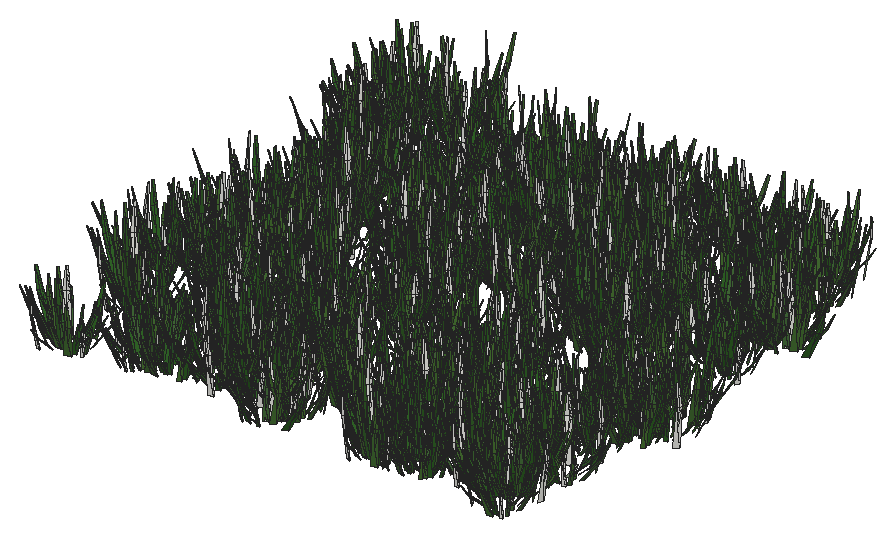
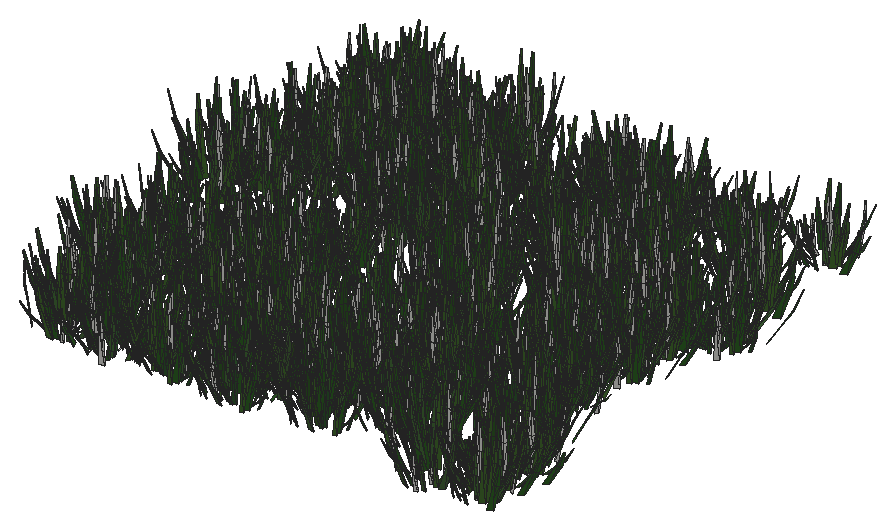
# SketchUp Ruby script. Lengths in inches.
U = 1.inch
M = Sketchup.active_model
def pt(a) = Geom::Point3d.new(a.map { |v| v * U })
def face(e, loops, mat)
  f = e.add_face(loops[0].map { |a| pt(a) })
  loops[1..].each { |l| e.add_face(l.map { |a| pt(a) }).erase! }
  f.material = f.back_material = mat if mat
  f
end
# faces: each face lists its corners as indices into pts; further lists are holes
def faces(e, pts, list, mat = nil) = list.each { |f| face(e, (f[0].is_a?(Array) ? f : [f]).map { |l| l.map { |i| pts[i] } }, mat) }
# xy, xz, yz: faces in a plane at the given z, y or x. An outline is a flat list of corners, or four numbers for a rectangle; further outlines are holes
def ring(l) = l.size == 4 ? [[l[0], l[1]], [l[2], l[1]], [l[2], l[3]], [l[0], l[3]]] : l.each_slice(2).to_a
def flat(e, list, mat, &to3) = list.each { |f| face(e, (f[0].is_a?(Array) ? f : [f]).map { |l| ring(l).map { |u, v| to3.(u, v) } }, mat) }
def xy(e, z, list, mat = nil) = flat(e, list, mat) { |x, y| [x, y, z] }
def xz(e, y, list, mat = nil) = flat(e, list, mat) { |x, z| [x, y, z] }
def yz(e, x, list, mat = nil) = flat(e, list, mat) { |y, z| [x, y, z] }
def lines(e, pts, list) = list.each { |a, b| e.add_line(pt(pts[a]), pt(pts[b])) }
# prism: a flat outline (further loops are holes) pulled along v
def prism(e, loops, v, mat = nil)
  f = face(e, loops, mat); d = Geom::Vector3d.new(v.map { |x| x * U })
  f.pushpull(f.normal.samedirection?(d) ? d.length : -d.length)
end
def box(e, o, s, mat = nil) = prism(e, [[o, [o[0] + s[0], o[1], o[2]], [o[0] + s[0], o[1] + s[1], o[2]], [o[0], o[1] + s[1], o[2]]]], [0, 0, s[2]], mat)
def at(x, y, z, deg = 0) = Geom::Transformation.translation(pt([x, y, z])) * Geom::Transformation.rotation(ORIGIN, Z_AXIS, deg.degrees)
def axes(o, x, y, z) = Geom::Transformation.new([*x, 0, *y, 0, *z, 0, *pt(o).to_a, 1])
def part(name) = M.definitions.add(name)
# library, detail: a bought-in or finely detailed component or shape, given as its bounding box
def library(name, o, s) = part(name).tap { |d| box(d.entities, o, s) }
def detail(e, o, s) = box(e.add_group.entities, o, s)
def put(e, d, t, mat = nil) = e.add_instance(d, t).tap { |i| i.material = mat if mat }
def group(e, t, mat = nil) = e.add_group.tap { |g| g.transformation = t; g.material = mat if mat }.entities
root = M.entities
M.materials.add("Material1").color = [58, 110, 58]
M.materials.add("Material10").color = [48, 100, 38]
M.materials.add("Material3").color = [68, 110, 58]
M.materials.add("Material4").color = [48, 90, 38]
M.materials.add("Material5").color = [68, 110, 48]
M.materials.add("Material6").color = [48, 90, 48]
M.materials.add("Material8").color = [58, 90, 38]
M.materials.add("Material9").color = [68, 100, 58]
c1 = part("grass00")
p = [[-0.6875,0.15,0],[-0.56,0.08,5.52],[-0.04,0.03,2.76],[0.48,-0.02,0],[0.35,-0.02,5.52],[-0.1,-0.14,5.52],
  [-0.12,0.65,8.37],[-0.42,0.65,8.37]]
faces(c1.entities,p,[[0,1,2,3],[3,2,4],[1,5,2],[5,4,2],[1,6,5],[4,5,6],[7,6,1]])
c2 = part("Group16\#1")
put(c2.entities,c1,axes([1.44,-0.61,-0.01],[0.05352,0.12609,0],[-0.10704,0.04543,0.07239],[0.06664,-0.02828,0.11628]),"Material6")
put(c2.entities,c1,axes([0.76,-0.15,-0.01],[0.04676,0.24062,0],[-0.23162,0.04501,0.06642],[0.0652,-0.01267,0.23595]),"Material3")
put(c2.entities,c1,axes([0.79,0.01,-0.01],[-0.00606,0.34651,0],[-0.34381,-0.00602,0.0432],[0.04319,0.00076,0.34386]))
put(c2.entities,c1,axes([1,0.23,-0.01],[-0.07192,0.31144,0],[-0.28722,-0.06632,0.1236],[0.12043,0.02781,0.29478]),"Material5")
put(c2.entities,c1,axes([1.66,0.77,-0.01],[-0.13828,0.29651,0],[-0.21551,-0.1005,0.22471],[0.20365,0.09498,0.23779]),"Material10")
put(c2.entities,c1,axes([0.6875,0.52,-0.01],[-0.18126,0.24051,0],[-0.22746,-0.17142,0.09788],[0.07817,0.05891,0.28481]),"Material5")
put(c2.entities,c1,axes([0.68,0.78,-0.01],[-0.215,0.18688,0],[-0.12385,-0.14248,0.21334],[0.13995,0.16101,0.18878]),"Material3")
put(c2.entities,c1,axes([0.56,1,-0.01],[-0.13756,0.07624,0],[-0.06159,-0.11112,0.0927],[0.04494,0.08108,0.12705]),"Material5")
put(c2.entities,c1,axes([0.2,0.64,-0.01],[-0.23729,0.07254,0],[-0.05711,-0.18681,0.153],[0.04473,0.14632,0.19535]),"Material10")
put(c2.entities,c1,axes([0.0625,0.72,-0.01],[-0.28874,0.02525,0],[-0.02179,-0.24916,0.14647],[0.01276,0.14591,0.25012]),"Material3")
put(c2.entities,c1,axes([-0.08,0.62,-0.01],[-0.34089,-0.04187,0],[0.03255,-0.26504,0.216],[-0.02633,0.21439,0.26703]),"Material10")
put(c2.entities,c1,axes([-0.34,0.98,-0.01],[-0.14314,-0.0493,0],[0.04397,-0.12769,0.06843],[-0.02228,0.0647,0.13505]),"Material10")
put(c2.entities,c1,axes([-0.87,1.45,-0.01],[-0.23488,-0.14114,0],[0.13761,-0.22901,0.06087],[-0.03135,0.05217,0.26717]))
put(c2.entities,c1,axes([-0.72,0.77,-0.01],[-0.14208,-0.13251,0],[0.07209,-0.0773,0.16301],[-0.11118,0.11922,0.1057]),"Material10")
put(c2.entities,c1,axes([-0.62,0.43,-0.01],[-0.14845,-0.21203,0],[0.18654,-0.13061,0.12304],[-0.10079,0.07057,0.22772]),"Material3")
put(c2.entities,c1,axes([-0.68,0.29,-0.01],[-0.13639,-0.32136,0],[0.31723,-0.13464,0.05579],[-0.05136,0.0218,0.34462]),"Material4")
put(c2.entities,c1,axes([-0.64,0.125,-0.01],[-0.0458,-0.23569,0],[0.22124,-0.043,0.08276],[-0.08124,0.01579,0.22538]),"Material1")
put(c2.entities,c1,axes([-1.6,-0.03,-0.01],[0.00576,-0.32897,0],[0.27526,0.00482,0.18018],[-0.18015,-0.00315,0.2753]),"Material5")
put(c2.entities,c1,axes([-1.36,-0.31,-0.01],[0.05718,-0.24765,0],[0.18172,0.04196,0.17267],[-0.16825,-0.03885,0.1865]),"Material10")
put(c2.entities,c1,axes([-1.54,-0.72,-0.01],[0.06537,-0.14017,0],[0.13555,0.06321,0.03939],[-0.0357,-0.01665,0.14956]))
put(c2.entities,c1,axes([-1.19,-0.9,-0.01],[0.09597,-0.12735,0],[0.11214,0.08451,0.07557],[-0.06035,-0.04548,0.14042]),"Material9")
put(c2.entities,c1,axes([-0.47,-0.54,-0.01],[0.11588,-0.10072,0],[0.0618,0.0711,0.12124],[-0.07953,-0.0915,0.0942]))
put(c2.entities,c1,axes([-0.47,-0.84,-0.01],[0.11927,-0.0661,0],[0.06603,0.11913,0.00646],[-0.00313,-0.00565,0.13621]),"Material5")
put(c2.entities,c1,axes([-0.38,-1.24,-0.01],[0.28037,-0.08571,0],[0.0618,0.20215,0.20315],[-0.05939,-0.19428,0.21139]),"Material9")
put(c2.entities,c1,axes([-0.06,-0.66,-0.01],[0.22719,-0.01987,0],[0.01247,0.14255,0.17758],[-0.01547,-0.17691,0.1431]),"Material8")
put(c2.entities,c1,axes([0.11,-0.89,-0.01],[0.14882,0.01828,0],[-0.01058,0.08611,0.12229],[0.01491,-0.12138,0.08676]),"Material6")
put(c2.entities,c1,axes([0.25,-0.72,-0.01],[0.20481,0.07053,0],[-0.06206,0.18022,0.10291],[0.03351,-0.0973,0.1906]),"Material6")
put(c2.entities,c1,axes([0.85,-1.42,-0.01],[0.16481,0.09904,0],[-0.09472,0.15762,0.05616],[0.02893,-0.04814,0.18389]),"Material5")
put(c2.entities,c1,axes([1.01,-1.09,-0.01],[0.21858,0.20385,0],[-0.17495,0.1876,0.15339],[0.10462,-0.11218,0.25652]),"Material10")
put(c2.entities,c1,axes([1.01,-0.71,-0.01],[0.08733,0.12473,0],[-0.06445,0.04512,0.13037],[0.1068,-0.07477,0.07867]),"Material6")
c3 = part("Group15\#1")
put(c3.entities,c2,at(0,0,0))
c4 = part("3darcstudiotree_grass00\#1")
put(c4.entities,c3,at(0,0,0))
put(root,c4,axes([268.09,130.14,0.25],[-0.53907,0.64308,0],[-0.93753,-0.5414,-0.02835],[-0.02982,-0.01722,1.46355]))
put(root,c4,axes([281.08,130.79,0.25],[0.67366,-0.68964,0],[0.84387,0.56787,-0.02965],[0.02907,0.01957,1.3715]))
put(root,c4,axes([290.375,131.09,0.25],[0.82276,0.36765,0],[-0.44369,0.68403,-0.02125],[-0.01422,0.02192,1.32121]))
put(root,c4,axes([272.48,131.14,0.25],[0.48793,0.72469,0],[-0.84905,0.39382,-0.02391],[-0.03201,0.01485,1.49173]))
put(root,c4,axes([287.89,131.01,0.25],[-0.6673,0.6871,0],[-0.74518,-0.49856,-0.02131],[-0.03285,-0.02198,1.8955]))
put(root,c4,axes([273.8125,131.37,0.25],[1.07141,0.38411,0],[-0.37972,0.72966,-0.02193],[-0.01335,0.02566,1.47013]))
put(root,c4,axes([296.6,131.16,0.25],[-0.24708,0.99531,0],[-0.9694,-0.16578,-0.03296],[-0.04602,-0.00787,1.411]))
put(root,c4,axes([290.92,131.76,0.25],[0.97736,0.04597,0],[-0.06009,0.88009,-0.02759],[-0.00232,0.03401,1.57942]))
put(root,c4,axes([281.9,132.04,0.25],[-0.01259,0.75713,0],[-1.00873,-0.01155,-0.02407],[-0.03563,-0.00041,1.49365]))
put(root,c4,axes([294.86,132.42,0.25],[1.04278,0.03697,0],[-0.04973,0.96637,-0.01987],[-0.00107,0.02079,1.47043]))
put(root,c4,axes([276.8,132.08,0.25],[-1.15536,0.20169,0],[-0.23741,-0.93689,-0.01674],[-0.00542,-0.02139,1.81501]))
put(root,c4,axes([278.76,132.28,0.25],[-1.14207,-0.30095,0],[0.33878,-0.88568,-0.0262],[0.00965,-0.02522,1.36239]))
put(root,c4,axes([293.48,132.32,0.25],[-0.89403,0.3818,0],[-0.42011,-0.6777,-0.01759],[-0.01685,-0.02718,1.92222]))
put(root,c4,axes([296.15,132.59,0.25],[-0.78578,-0.85776,0],[0.88481,-0.55839,-0.02],[0.02549,-0.01608,1.779]))
put(root,c4,axes([277.31,133.39,0.25],[1.01426,-0.49886,0],[0.46228,0.64748,-0.02001],[0.01932,0.02706,1.71774]))
put(root,c4,axes([287.05,133.4375,0.25],[0.21033,-0.77468,0],[1.11625,0.20878,-0.02216],[0.02884,0.00539,1.52603]))
put(root,c4,axes([279.79,133.33,0.25],[-0.64583,-0.8636,0],[0.92417,-0.47612,-0.02087],[0.02583,-0.01331,1.58468]))
put(root,c4,axes([278.83,133.83,0.25],[0.95,0.05182,0],[-0.07465,0.94272,-0.01423],[-0.0015,0.01897,1.83161]))
put(root,c4,axes([289.43,133.89,0.25],[1.00049,0.45654,0],[-0.52748,0.79633,-0.0244],[-0.01411,0.0213,1.31386]))
put(root,c4,axes([288.54,134.26,0.25],[-0.93177,-0.64283,0],[0.5837,-0.58286,-0.01701],[0.02329,-0.02326,1.95649]))
put(root,c4,axes([270.44,134.78,0.25],[-0.98266,0.19037,0],[-0.20775,-0.73875,-0.0198],[-0.00727,-0.02586,1.47686]))
put(root,c4,axes([283.35,134.95,0.25],[0.02763,0.80603,0],[-1.11819,0.02641,-0.02239],[-0.03678,0.00087,1.83839]))
put(root,c4,axes([294.7,135.03,0.25],[-0.07113,0.78649,0],[-1.00905,-0.06286,-0.02554],[-0.04133,-0.00258,1.64241]))
put(root,c4,axes([275.19,135.01,0.25],[-0.15456,0.818,0],[-0.95893,-0.12482,-0.01794],[-0.02914,-0.00379,1.59592]))
put(root,c4,axes([287.54,135.73,0.25],[0.74168,-0.7433,0],[0.8948,0.61509,-0.01649],[0.01966,0.01351,1.79785]))
put(root,c4,axes([285.71,135.64,0.25],[1.16836,-0.073,0],[0.07339,0.80916,-0.02417],[0.00336,0.03702,1.80918]))
put(root,c4,axes([290.68,135.67,0.25],[0.16151,-0.86236,0],[1.11997,0.1445,-0.01704],[0.02682,0.00346,1.80481]))
put(root,c4,axes([293.51,135.55,0.25],[-0.84719,0.42792,0],[-0.59614,-0.81305,-0.01391],[-0.0109,-0.01487,1.7292]))
put(root,c4,axes([296.86,135.72,0.25],[-0.20555,0.89132,0],[-1.21308,-0.19272,-0.01652],[-0.01977,-0.00314,1.50529]))
put(root,c4,axes([294.62,135.84,0.25],[-0.83493,0.34235,0],[-0.4809,-0.80796,-0.03032],[-0.01856,-0.03119,1.50108]))
put(root,c4,axes([268.17,135.81,0.25],[-0.71425,0.8071,0],[-0.94598,-0.57671,-0.02364],[-0.03147,-0.01919,1.93862]))
put(root,c4,axes([276.57,136,0.25],[-1.12239,-0.08801,0],[0.1009,-0.88648,-0.03137],[0.00364,-0.03196,1.3228]))
put(root,c4,axes([279.55,136.25,0.25],[0.63983,0.86869,0],[-0.81658,0.41433,-0.02868],[-0.03873,0.01965,1.51486]))
put(root,c4,axes([275.14,136.92,0.25],[-1.23081,-0.22961,0],[0.22785,-0.84141,-0.03373],[0.00949,-0.03505,1.33323]))
put(root,c4,axes([273.9,137.4,0.25],[-0.00132,-0.89623,0],[1.27155,-0.00129,-0.02113],[0.02355,-0.00002,1.41674]))
put(root,c4,axes([279.91,137.25,0.25],[0.60365,0.68423,0],[-0.80016,0.48631,-0.01948],[-0.02732,0.0166,1.72408]))
put(root,c4,axes([295.13,137.45,0.25],[-0.40192,0.84497,0],[-1.13388,-0.37155,-0.02576],[-0.03011,-0.00987,1.53201]))
put(root,c4,axes([285.43,138.54,0.25],[0.03803,-1.04243,0],[1.12016,0.02816,-0.01983],[0.02669,0.00067,1.50947]))
put(root,c4,axes([287.3,138.57,0.25],[-0.13032,-0.91195,0],[1.13894,-0.11213,-0.02638],[0.033,-0.00325,1.44452]))
put(root,c4,axes([280.06,138.61,0.25],[0.91623,0.64019,0],[-0.77498,0.76409,-0.01247],[-0.01243,0.01226,1.86292]))
put(root,c4,axes([278.48,138.51,0.25],[0.20989,0.98932,0],[-0.91705,0.13403,-0.02162],[-0.03023,0.00442,1.32159]))
put(root,c4,axes([271.8125,138.87,0.25],[0.98513,-0.24233,0],[0.2644,0.74045,-0.03127],[0.01421,0.0398,1.48816]))
put(root,c4,axes([296.52,138.85,0.25],[-0.88603,-0.29285,0],[0.47173,-0.98323,-0.01803],[0.0095,-0.01979,1.81493]))
put(root,c4,axes([289.14,139.67,0.25],[0.39466,-0.92638,0],[0.88692,0.2603,-0.02361],[0.03123,0.00917,1.32009]))
put(root,c4,axes([272.48,139.65,0.25],[0.17834,0.988,0],[-1.21851,0.15152,-0.01905],[-0.02401,0.00299,1.57029]))
put(root,c4,axes([290.37,140.1,0.25],[1.04138,0.00688,0],[-0.00783,0.81623,-0.01492],[-0.00022,0.02319,1.84219]))
put(root,c4,axes([266.77,139.96,0.25],[-1.10511,-0.09351,0],[0.12142,-0.98854,-0.03002],[0.00407,-0.0331,1.59842]))
put(root,c4,axes([293.64,140.56,0.25],[-0.19314,-0.90821,0],[0.93219,-0.13657,-0.01992],[0.03322,-0.00487,1.60321]))
put(root,c4,axes([276.69,140.63,0.25],[-0.41592,-0.90792,0],[1.20282,-0.37959,-0.02869],[0.02934,-0.00926,1.40786]))
put(root,c4,axes([297.02,140.85,0.25],[1.04863,0.59418,0],[-0.60818,0.73943,-0.02215],[-0.02194,0.02667,1.8946]))
put(root,c4,axes([267.49,140.96,0.25],[1.03267,0.30611,0],[-0.42943,0.99799,-0.02984],[-0.01222,0.02841,1.55474]))
put(root,c4,axes([275,140.7,0.25],[-0.90293,0.73238,0],[-0.69177,-0.58754,-0.01484],[-0.01942,-0.0165,1.85373]))
put(root,c4,axes([287.25,141.14,0.25],[1.21974,-0.24702,0],[0.24172,0.82225,-0.01844],[0.0078,0.02655,1.82062]))
put(root,c4,axes([282.53,141.32,0.25],[-0.55601,0.81305,0],[-1.0854,-0.51135,-0.03094],[-0.02916,-0.01374,1.35284]))
put(root,c4,axes([269.13,141.43,0.25],[-0.18187,0.76439,0],[-1.22651,-0.20104,-0.01512],[-0.02206,-0.00362,1.85999]))
put(root,c4,axes([295.15,142.02,0.25],[1.16526,-0.01071,0],[0.01084,0.81226,-0.01976],[0.00031,0.02293,1.36845]))
put(root,c4,axes([288.64,141.83,0.25],[-0.97391,-0.22874,0],[0.24921,-0.73098,-0.03071],[0.01267,-0.03717,1.38702]))
put(root,c4,axes([287.09,142.54,0.25],[1.04221,-0.36679,0],[0.41999,0.82212,-0.02583],[0.01581,0.03095,1.68703]))
put(root,c4,axes([296.65,142.19,0.25],[-0.43733,0.86277,0],[-0.88377,-0.30861,-0.02216],[-0.03542,-0.01237,1.66252]))
put(root,c4,axes([281.19,142.51,0.25],[-0.34265,-0.71824,0],[0.84601,-0.27805,-0.01359],[0.02323,-0.00763,1.67314]))
put(root,c4,axes([298.27,142.38,0.25],[-1.16875,-0.4714,0],[0.51721,-0.88339,-0.01545],[0.01039,-0.01775,1.8215]))
put(root,c4,axes([276.61,142.53,0.25],[-0.4531,0.70916,0],[-0.81981,-0.36084,-0.02105],[-0.03771,-0.0166,1.88169]))
put(root,c4,axes([273.82,143.29,0.25],[0.67947,-0.60049,0],[0.75522,0.58869,-0.02466],[0.02767,0.02157,1.59511]))
put(root,c4,axes([270.6,143.38,0.25],[0.01927,-0.98763,0],[1.28715,0.0173,-0.02796],[0.03462,0.00047,1.59394]))
put(root,c4,axes([295.55,143.07,0.25],[-0.63139,0.7109,0],[-0.77977,-0.4771,-0.0238],[-0.03163,-0.01935,1.59896]))
put(root,c4,axes([268.75,143.42,0.25],[-0.75617,0.48465,0],[-0.65878,-0.70809,-0.02049],[-0.01652,-0.01776,1.42185]))
put(root,c4,axes([279.64,143.76,0.25],[-0.96266,-0.0089,0],[0.0103,-0.76764,-0.02017],[0.00043,-0.03215,1.77597]))
put(root,c4,axes([283.04,143.68,0.25],[-0.68998,0.78183,0],[-0.74383,-0.45223,-0.02032],[-0.02946,-0.01791,1.65635]))
put(root,c4,axes([274.03,144.72,0.25],[1.04663,-0.61826,0],[0.54759,0.6386,-0.02041],[0.0245,0.02857,1.95445]))
put(root,c4,axes([270.5,145.01,0.25],[-0.37741,-0.85263,0],[0.87967,-0.26825,-0.02344],[0.03148,-0.0096,1.34096]))
put(root,c4,axes([297.82,144.79,0.25],[-0.85067,0.58749,0],[-0.79131,-0.78933,-0.01948],[-0.01821,-0.01816,1.80807]))
put(root,c4,axes([287.87,145.05,0.25],[-0.29839,0.74315,0],[-0.85367,-0.23613,-0.02384],[-0.04548,-0.01258,1.80943]))
put(root,c4,axes([268.89,145.85,0.25],[-1.21628,0.04219,0],[-0.04215,-0.83708,-0.02048],[-0.00169,-0.0336,1.99696]))
put(root,c4,axes([280.41,146.32,0.25],[-1.0506,0.1923,0],[-0.25327,-0.95326,-0.02531],[-0.00821,-0.03089,1.77094]))
put(root,c4,axes([269.6,146.91,0.25],[0.98205,0.32033,0],[-0.38236,0.80754,-0.02634],[-0.01461,0.03085,1.58474]))
put(root,c4,axes([289.15,147.41,0.25],[0.93743,0.58404,0],[-0.68609,0.75863,-0.02233],[-0.02309,0.02554,1.9689]))
put(root,c4,axes([272.52,147.47,0.25],[-1.05565,-0.35252,0],[0.37885,-0.78155,-0.02256],[0.01288,-0.02658,1.55256]))
put(root,c4,axes([290.99,147.63,0.25],[0.04648,1.04807,0],[-1.26019,0.0385,-0.03073],[-0.03624,0.00111,1.48809]))
put(root,c4,axes([278.49,147.77,0.25],[-1.1416,-0.50884,0],[0.50806,-0.78524,-0.02099],[0.01379,-0.02131,1.49075]))
put(root,c4,axes([279.87,148.1,0.25],[1.01468,-0.04576,0],[0.05371,0.82049,-0.02262],[0.002,0.03055,1.6131]))
put(root,c4,axes([270.28,148.18,0.25],[-1.0469,-0.18453,0],[0.24055,-0.94015,-0.02543],[0.00733,-0.02866,1.60712]))
put(root,c4,axes([277.28,148.4,0.25],[-0.45666,0.64648,0],[-0.9789,-0.47635,-0.01566],[-0.01927,-0.00938,1.61828]))
put(root,c4,axes([275.87,148.89,0.25],[0.46409,-0.72665,0],[1.0563,0.46475,-0.01977],[0.02609,0.01148,1.78562]))
put(root,c4,axes([269.75,148.95,0.25],[0.82703,-0.66636,0],[0.66302,0.56689,-0.02978],[0.03123,0.0267,1.43312]))
put(root,c4,axes([290.65,149.02,0.25],[1.07013,0.57514,0],[-0.63913,0.81923,-0.02279],[-0.01983,0.02542,1.88252]))
put(root,c4,axes([283.09,149.61,0.25],[-0.12772,-0.94069,0],[1.04105,-0.09738,-0.02839],[0.0355,-0.00332,1.31807]))
put(root,c4,axes([291.6,149.6,0.25],[1.0301,0.12261,0],[-0.13856,0.80197,-0.02285],[-0.00447,0.02587,1.34478]))
put(root,c4,axes([288.39,149.73,0.25],[0.0857,-0.75553,0],[0.98417,0.0769,-0.01523],[0.03053,0.00239,1.99019]))
put(root,c4,axes([287.25,149.62,0.25],[0.60972,0.76491,0],[-1.05055,0.57689,-0.02773],[-0.02774,0.01523,1.51065]))
put(root,c4,axes([290.29,149.53,0.25],[0.50923,0.96621,0],[-0.88369,0.32084,-0.02724],[-0.03888,0.01412,1.50258]))
put(root,c4,axes([296.86,149.65,0.25],[-0.81312,-0.35167,0],[0.49817,-0.79352,-0.0201],[0.0112,-0.01784,1.30027]))
put(root,c4,axes([270.55,150.08,0.25],[0.81917,-0.50902,0],[0.69547,0.77104,-0.01707],[0.01728,0.01916,1.96039]))
put(root,c4,axes([281.48,149.66,0.25],[-1.16872,-0.00836,0],[0.01032,-0.99435,-0.00939],[0.00013,-0.01237,1.9024]))
put(root,c4,axes([269.17,150.02,0.25],[0.69931,0.58263,0],[-0.8498,0.70267,-0.03194],[-0.02573,0.02127,1.36388]))
put(root,c4,axes([295.25,150.72,0.25],[1.20567,0.27719,0],[-0.34397,1.03067,-0.02222],[-0.0089,0.02668,1.93436]))
put(root,c4,axes([286.25,150.84,0.25],[-0.69806,-0.65492,0],[0.75287,-0.55282,-0.02762],[0.03461,-0.02541,1.68176]))
put(root,c4,axes([290.26,151.19,0.25],[0.83832,-0.32147,0],[0.3911,0.7026,-0.0238],[0.02048,0.0368,1.9133]))
put(root,c4,axes([288.93,150.88,0.25],[0.11246,1.02167,0],[-0.98674,0.07482,-0.02215],[-0.0317,0.0024,1.42375]))
put(root,c4,axes([293.48,151.02,0.25],[-0.53893,0.846,0],[-1.11511,-0.48937,-0.01892],[-0.01942,-0.00852,1.46501]))
put(root,c4,axes([270.96,151.2,0.25],[0.5099,0.89174,0],[-0.93685,0.36904,-0.01135],[-0.01786,0.00703,1.80626]))
put(root,c4,axes([268.89,152.45,0.25],[0.58458,-0.74588,0],[0.82467,0.44526,-0.01966],[0.02752,0.01486,1.64285]))
put(root,c4,axes([278.54,152.18,0.25],[-0.41748,0.72425,0],[-0.99279,-0.39424,-0.02774],[-0.03217,-0.01277,1.41462]))
put(root,c4,axes([276.62,152.21,0.25],[-0.48847,0.79594,0],[-1.13522,-0.47995,-0.01882],[-0.01964,-0.0083,1.49212]))
put(root,c4,axes([274.76,152.71,0.25],[-0.4468,-0.74651,0],[1.00463,-0.41423,-0.01655],[0.02363,-0.00974,1.78815]))
put(root,c4,axes([286.1,153.33,0.25],[0.58175,-0.8795,0],[0.91077,0.41502,-0.02765],[0.03587,0.01634,1.53783]))
put(root,c4,axes([270.62,153.35,0.25],[1.12554,0.27273,0],[-0.28923,0.82228,-0.03197],[-0.01194,0.03395,1.37583]))
put(root,c4,axes([296.43,153.46,0.25],[0.38138,0.89444,0],[-0.93044,0.27331,-0.0171],[-0.03017,0.00886,1.84743]))
put(root,c4,axes([281.35,153.43,0.25],[-0.41167,0.67471,0],[-0.96597,-0.40603,-0.03106],[-0.0339,-0.01425,1.32443]))
put(root,c4,axes([294.61,153.89,0.25],[0.92791,-0.50784,0],[0.64696,0.81436,-0.02666],[0.01858,0.02339,1.48784]))
put(root,c4,axes([284.55,153.88,0.25],[0.60411,-0.79044,0],[0.78393,0.41274,-0.01781],[0.02433,0.01281,1.50117]))
put(root,c4,axes([290.59,153.73,0.25],[0.75774,0.45617,0],[-0.52933,0.60573,-0.02439],[-0.02554,0.02923,1.60766]))
put(root,c4,axes([297.62,153.97,0.25],[0.5985,-0.67578,0],[0.98245,0.59941,-0.0227],[0.02414,0.01473,1.60931]))
put(root,c4,axes([273.74,153.9,0.25],[0.79627,0.65567,0],[-0.71624,0.59922,-0.02475],[-0.02794,0.02337,1.62992]))
put(root,c4,axes([274.78,153.98,0.25],[0.17811,0.99351,0],[-0.9394,0.11602,-0.01524],[-0.03015,0.00372,1.90022]))
put(root,c4,axes([273.77,154.48,0.25],[1.19487,0.08138,0],[-0.07553,0.76404,-0.01884],[-0.00229,0.02315,1.37151]))
put(root,c4,axes([281.88,154.72,0.25],[0.93297,-0.65602,0],[0.76381,0.74833,-0.02128],[0.01868,0.0183,1.60475]))
put(root,c4,axes([267.93,154.67,0.25],[-1.02564,-0.16376,0],[0.18604,-0.80269,-0.01319],[0.00445,-0.01922,1.76124]))
put(root,c4,axes([277.98,155.08,0.25],[1.15701,-0.19315,0],[0.2232,0.92103,-0.02659],[0.00704,0.02903,1.51897]))
put(root,c4,axes([284.97,154.68,0.25],[-1.10882,0.55302,0],[-0.48301,-0.66717,-0.02116],[-0.01735,-0.02397,1.49339]))
put(root,c4,axes([279.83,155.32,0.25],[-1.27134,0.01132,0],[-0.01287,-0.99645,-0.01941],[-0.00033,-0.02588,1.92834]))
put(root,c4,axes([277.11,155.91,0.25],[0.0754,-0.91723,0],[1.27705,0.07232,-0.02398],[0.02445,0.00138,1.30813]))
put(root,c4,axes([275.07,155.72,0.25],[-0.97907,-0.67112,0],[0.76655,-0.77039,-0.02974],[0.02124,-0.02135,1.35064]))
put(root,c4,axes([278.17,156.23,0.25],[0.06446,-0.92211,0],[1.06917,0.05149,-0.02273],[0.03185,0.00153,1.50351]))
put(root,c4,axes([293.96,156.05,0.25],[-0.7945,-0.59925,0],[0.81455,-0.74398,-0.02206],[0.0199,-0.01818,1.62457]))
put(root,c4,axes([288.64,156.31,0.25],[-0.03397,-0.83384,0],[0.91245,-0.02561,-0.02047],[0.03733,-0.00105,1.66543]))
put(root,c4,axes([267.84,156.31,0.25],[-0.30667,-0.85944,0],[0.90928,-0.22352,-0.01669],[0.03071,-0.00755,1.82011]))
put(root,c4,axes([287.46,156.17,0.25],[0.08868,0.74456,0],[-1.0596,0.08695,-0.01511],[-0.02758,0.00226,1.95375]))
put(root,c4,axes([295.375,156.46,0.25],[0.39113,0.83248,0],[-1.19652,0.38728,-0.01645],[-0.02102,0.0068,1.76201]))
put(root,c4,axes([279.4375,157.51,0.25],[0.88313,-0.5796,0],[0.73666,0.77324,-0.01988],[0.02039,0.0214,1.96304]))
put(root,c4,axes([283.39,157.48,0.25],[-0.40474,-0.99037,0],[0.94061,-0.26482,-0.01224],[0.0231,-0.0065,1.97883]))
put(root,c4,axes([285.5,157.51,0.25],[-0.19194,-0.96358,0],[1.13233,-0.15538,-0.0168],[0.0224,-0.00307,1.55067]))
put(root,c4,axes([266.49,157.36,0.25],[-0.68531,0.71907,0],[-0.89492,-0.58757,-0.0328],[-0.02989,-0.01962,1.32564]))
put(root,c4,axes([274.95,158.33,0.25],[0.73142,0.45159,0],[-0.55142,0.61527,-0.0148],[-0.01846,0.02059,1.93047]))
put(root,c4,axes([293.6,158.18,0.25],[-0.95322,-0.32431,0],[0.44192,-0.89482,-0.01809],[0.00873,-0.01768,1.4829]))
put(root,c4,axes([284.12,158.46,0.25],[-0.25986,-1.02981,0],[1.17432,-0.20414,-0.02019],[0.02797,-0.00486,1.69814]))
put(root,c4,axes([268.08,158.3125,0.25],[-1.11715,-0.19884,0],[0.22044,-0.85322,-0.03168],[0.00925,-0.0358,1.46389]))
put(root,c4,axes([272.77,158.58,0.25],[-0.88558,-0.6265,0],[0.61255,-0.59649,-0.02002],[0.01793,-0.01746,1.30322]))
put(root,c4,axes([283.28,158.88,0.25],[-0.86549,-0.80042,0],[0.87843,-0.65434,-0.02493],[0.02251,-0.01677,1.43253]))
put(root,c4,axes([295.97,158.74,0.25],[-0.23853,0.95506,0],[-1.01193,-0.17411,-0.02464],[-0.04194,-0.00722,1.79662]))
put(root,c4,axes([281.82,159.03,0.25],[-0.60981,-0.62703,0],[0.7521,-0.50389,-0.02577],[0.03248,-0.02176,1.56591]))
put(root,c4,axes([279.72,158.88,0.25],[-0.987,-0.0893,0],[0.12647,-0.96294,-0.01401],[0.00225,-0.01714,1.72979]))
put(root,c4,axes([266.74,159.49,0.25],[-0.71016,0.58255,0],[-0.84104,-0.70632,-0.01852],[-0.01637,-0.01375,1.50457]))
put(root,c4,axes([291.8,159.93,0.25],[-1.02282,-0.44061,0],[0.49107,-0.78532,-0.02416],[0.01513,-0.0242,1.4491]))
put(root,c4,axes([284.46,160.26,0.25],[0.98816,-0.32737,0],[0.37679,0.7835,-0.02611],[0.01369,0.02847,1.43783]))
put(root,c4,axes([278.1,160.28,0.25],[-0.95876,-0.4118,0],[0.50951,-0.81721,-0.02021],[0.01606,-0.02576,1.91641]))
put(root,c4,axes([289.11,160.23,0.25],[-0.17865,0.84574,0],[-1.04848,-0.15257,-0.02601],[-0.03998,-0.00582,1.66111]))
put(root,c4,axes([294.89,160.98,0.25],[0.07043,-0.84147,0],[1.09097,0.06291,-0.0172],[0.02632,0.00152,1.67763]))
put(root,c4,axes([287.73,161.04,0.25],[-1.26931,0.09939,0],[-0.08571,-0.75407,-0.02738],[-0.00461,-0.04056,1.63584]))
put(root,c4,axes([269.79,161.34,0.25],[-0.33921,-1.0236,0],[1.14484,-0.26135,-0.02011],[0.03211,-0.00733,1.9663]))
put(root,c4,axes([283.21,161.22,0.25],[-1.12582,-0.22526,0],[0.23567,-0.81144,-0.01967],[0.00737,-0.02538,1.60841]))
put(root,c4,axes([291.64,161.49,0.25],[0.98143,-0.05451,0],[0.06758,0.83814,-0.02393],[0.00238,0.02949,1.50627]))
put(root,c4,axes([266.56,161.17,0.25],[-0.40449,0.78017,0],[-0.96003,-0.3429,-0.01574],[-0.02302,-0.00822,1.66349]))
